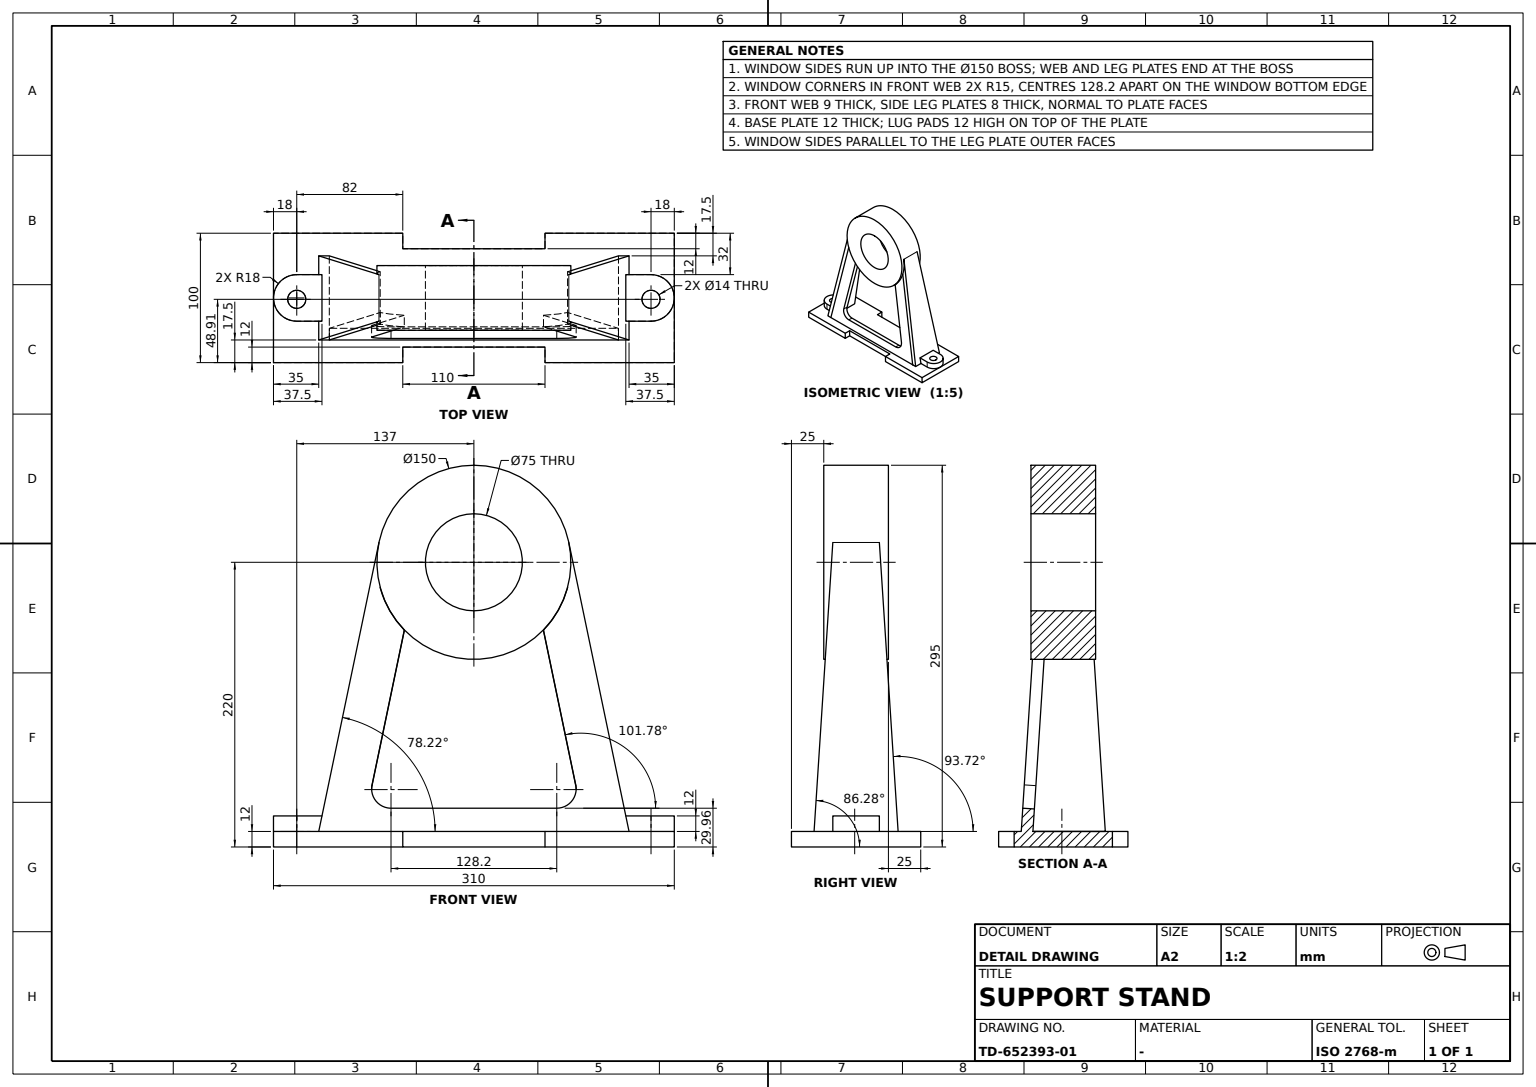
ISO-10303-21;
HEADER;
FILE_DESCRIPTION((''),'2;1');
FILE_NAME('','',(''),(''),'','','');
FILE_SCHEMA(('AUTOMOTIVE_DESIGN'));
ENDSEC;
DATA;
#1=APPLICATION_CONTEXT('');
#2=PRODUCT_CONTEXT('',#1,'mechanical');
#3=PRODUCT('','','',(#2));
#4=PRODUCT_DEFINITION_FORMATION('','',#3);
#5=PRODUCT_DEFINITION_CONTEXT('',#1,'design');
#6=PRODUCT_DEFINITION('','',#4,#5);
#7=PRODUCT_DEFINITION_SHAPE('','',#6);
#8=(LENGTH_UNIT()NAMED_UNIT(*)SI_UNIT(.MILLI.,.METRE.));
#9=(NAMED_UNIT(*)PLANE_ANGLE_UNIT()SI_UNIT($,.RADIAN.));
#10=(NAMED_UNIT(*)SI_UNIT($,.STERADIAN.)SOLID_ANGLE_UNIT());
#11=UNCERTAINTY_MEASURE_WITH_UNIT(LENGTH_MEASURE(0.005),#8,'distance_accuracy_value','');
#12=(GEOMETRIC_REPRESENTATION_CONTEXT(3)GLOBAL_UNCERTAINTY_ASSIGNED_CONTEXT((#11))GLOBAL_UNIT_ASSIGNED_CONTEXT((#8,#9,#10))REPRESENTATION_CONTEXT('',''));
#13=CARTESIAN_POINT('',(120.,32.5,0.));
#14=VERTEX_POINT('',#13);
#15=CARTESIAN_POINT('',(111.827821,32.5,0.));
#16=VERTEX_POINT('',#15);
#17=CARTESIAN_POINT('',(0.,32.5,0.));
#18=DIRECTION('',(-1.,0.,0.));
#19=VECTOR('',#18,1000.);
#20=LINE('',#17,#19);
#21=EDGE_CURVE('',#14,#16,#20,.T.);
#22=ORIENTED_EDGE('',*,*,#21,.F.);
#23=CARTESIAN_POINT('',(120.,18.,0.));
#24=VERTEX_POINT('',#23);
#25=CARTESIAN_POINT('',(120.,0.,0.));
#26=DIRECTION('',(0.,1.,0.));
#27=VECTOR('',#26,1000.);
#28=LINE('',#25,#27);
#29=EDGE_CURVE('',#24,#14,#28,.T.);
#30=ORIENTED_EDGE('',*,*,#29,.F.);
#31=CARTESIAN_POINT('',(137.,18.,0.));
#32=VERTEX_POINT('',#31);
#33=LINE('',#31,#19);
#34=EDGE_CURVE('',#32,#24,#33,.T.);
#35=ORIENTED_EDGE('',*,*,#34,.F.);
#36=CARTESIAN_POINT('',(155.,0.,0.));
#37=VERTEX_POINT('',#36);
#38=CARTESIAN_POINT('',(137.,0.,0.));
#39=DIRECTION('',(0.,0.,-1.));
#40=AXIS2_PLACEMENT_3D('',#38,#39,#18);
#41=CIRCLE('',#40,18.);
#42=EDGE_CURVE('',#37,#32,#41,.F.);
#43=ORIENTED_EDGE('',*,*,#42,.F.);
#44=CARTESIAN_POINT('',(155.,50.,0.));
#45=VERTEX_POINT('',#44);
#46=DIRECTION('',(0.,-1.,0.));
#47=VECTOR('',#46,1000.);
#48=LINE('',#36,#47);
#49=EDGE_CURVE('',#45,#37,#48,.T.);
#50=ORIENTED_EDGE('',*,*,#49,.F.);
#51=CARTESIAN_POINT('',(55.,50.,0.));
#52=VERTEX_POINT('',#51);
#53=CARTESIAN_POINT('',(0.,50.,0.));
#54=DIRECTION('',(1.,0.,0.));
#55=VECTOR('',#54,1000.);
#56=LINE('',#53,#55);
#57=EDGE_CURVE('',#52,#45,#56,.T.);
#58=ORIENTED_EDGE('',*,*,#57,.F.);
#59=CARTESIAN_POINT('',(55.,38.,0.));
#60=VERTEX_POINT('',#59);
#61=CARTESIAN_POINT('',(55.,0.,0.));
#62=LINE('',#61,#27);
#63=EDGE_CURVE('',#60,#52,#62,.T.);
#64=ORIENTED_EDGE('',*,*,#63,.F.);
#65=CARTESIAN_POINT('',(-55.,38.,0.));
#66=VERTEX_POINT('',#65);
#67=CARTESIAN_POINT('',(0.,38.,0.));
#68=LINE('',#67,#55);
#69=EDGE_CURVE('',#66,#60,#68,.T.);
#70=ORIENTED_EDGE('',*,*,#69,.F.);
#71=CARTESIAN_POINT('',(-55.,50.,0.));
#72=VERTEX_POINT('',#71);
#73=CARTESIAN_POINT('',(-55.,0.,0.));
#74=LINE('',#73,#47);
#75=EDGE_CURVE('',#72,#66,#74,.T.);
#76=ORIENTED_EDGE('',*,*,#75,.F.);
#77=CARTESIAN_POINT('',(-155.,50.,0.));
#78=VERTEX_POINT('',#77);
#79=EDGE_CURVE('',#78,#72,#56,.T.);
#80=ORIENTED_EDGE('',*,*,#79,.F.);
#81=CARTESIAN_POINT('',(-155.,0.,0.));
#82=VERTEX_POINT('',#81);
#83=LINE('',#81,#27);
#84=EDGE_CURVE('',#82,#78,#83,.T.);
#85=ORIENTED_EDGE('',*,*,#84,.F.);
#86=CARTESIAN_POINT('',(-137.,18.,0.));
#87=VERTEX_POINT('',#86);
#88=CARTESIAN_POINT('',(-137.,0.,0.));
#89=AXIS2_PLACEMENT_3D('',#88,#39,#18);
#90=CIRCLE('',#89,18.);
#91=EDGE_CURVE('',#82,#87,#90,.T.);
#92=ORIENTED_EDGE('',*,*,#91,.T.);
#93=CARTESIAN_POINT('',(-120.,18.,0.));
#94=VERTEX_POINT('',#93);
#95=CARTESIAN_POINT('',(0.,18.,0.));
#96=LINE('',#95,#55);
#97=EDGE_CURVE('',#87,#94,#96,.T.);
#98=ORIENTED_EDGE('',*,*,#97,.T.);
#99=CARTESIAN_POINT('',(-120.,32.5,0.));
#100=VERTEX_POINT('',#99);
#101=CARTESIAN_POINT('',(-120.,0.,0.));
#102=LINE('',#101,#27);
#103=EDGE_CURVE('',#94,#100,#102,.T.);
#104=ORIENTED_EDGE('',*,*,#103,.T.);
#105=CARTESIAN_POINT('',(-111.827821,32.5,0.));
#106=VERTEX_POINT('',#105);
#107=EDGE_CURVE('',#106,#100,#20,.T.);
#108=ORIENTED_EDGE('',*,*,#107,.F.);
#109=CARTESIAN_POINT('',(-111.827821,-32.5,0.));
#110=VERTEX_POINT('',#109);
#111=CARTESIAN_POINT('',(-111.827821,0.,0.));
#112=LINE('',#111,#47);
#113=EDGE_CURVE('',#106,#110,#112,.T.);
#114=ORIENTED_EDGE('',*,*,#113,.T.);
#115=CARTESIAN_POINT('',(-111.706184,-23.481048,0.));
#116=VERTEX_POINT('',#115);
#117=CARTESIAN_POINT('',(-111.369243,1.502014,0.));
#118=DIRECTION('',(0.013485569,0.999909066,0.));
#119=VECTOR('',#118,1000.);
#120=LINE('',#117,#119);
#121=EDGE_CURVE('',#110,#116,#120,.T.);
#122=ORIENTED_EDGE('',*,*,#121,.T.);
#123=CARTESIAN_POINT('',(111.706184,-23.481048,0.));
#124=VERTEX_POINT('',#123);
#125=CARTESIAN_POINT('',(0.,-23.481048,0.));
#126=LINE('',#125,#55);
#127=EDGE_CURVE('',#116,#124,#126,.T.);
#128=ORIENTED_EDGE('',*,*,#127,.T.);
#129=CARTESIAN_POINT('',(111.827821,-32.5,0.));
#130=VERTEX_POINT('',#129);
#131=CARTESIAN_POINT('',(111.369243,1.502014,0.));
#132=DIRECTION('',(-0.013485569,0.999909066,0.));
#133=VECTOR('',#132,1000.);
#134=LINE('',#131,#133);
#135=EDGE_CURVE('',#130,#124,#134,.T.);
#136=ORIENTED_EDGE('',*,*,#135,.F.);
#137=CARTESIAN_POINT('',(111.827821,0.,0.));
#138=LINE('',#137,#47);
#139=EDGE_CURVE('',#16,#130,#138,.T.);
#140=ORIENTED_EDGE('',*,*,#139,.F.);
#141=EDGE_LOOP('',(#22,#30,#35,#43,#50,#58,#64,#70,#76,#80,#85,#92,#98,#104,#108,#114,#122,#128,#136,#140));
#142=FACE_BOUND('',#141,.T.);
#143=CARTESIAN_POINT('',(0.,0.,0.));
#144=AXIS2_PLACEMENT_3D('',#143,#39,#18);
#145=PLANE('',#144);
#146=ADVANCED_FACE('',(#142),#145,.F.);
#147=CARTESIAN_POINT('',(-137.,-18.,12.));
#148=VERTEX_POINT('',#147);
#149=CARTESIAN_POINT('',(-137.,18.,12.));
#150=VERTEX_POINT('',#149);
#151=CARTESIAN_POINT('',(-137.,0.,12.));
#152=DIRECTION('',(0.,0.,1.));
#153=AXIS2_PLACEMENT_3D('',#151,#152,#54);
#154=CIRCLE('',#153,18.);
#155=EDGE_CURVE('',#148,#150,#154,.F.);
#156=ORIENTED_EDGE('',*,*,#155,.F.);
#157=CARTESIAN_POINT('',(-117.496972,-18.,12.));
#158=VERTEX_POINT('',#157);
#159=CARTESIAN_POINT('',(115.,-18.,12.));
#160=LINE('',#159,#19);
#161=EDGE_CURVE('',#158,#148,#160,.T.);
#162=ORIENTED_EDGE('',*,*,#161,.F.);
#163=CARTESIAN_POINT('',(-117.496972,18.,12.));
#164=VERTEX_POINT('',#163);
#165=CARTESIAN_POINT('',(-117.496972,0.,12.));
#166=LINE('',#165,#47);
#167=EDGE_CURVE('',#164,#158,#166,.T.);
#168=ORIENTED_EDGE('',*,*,#167,.F.);
#169=CARTESIAN_POINT('',(137.,18.,12.));
#170=LINE('',#169,#55);
#171=EDGE_CURVE('',#150,#164,#170,.T.);
#172=ORIENTED_EDGE('',*,*,#171,.F.);
#173=EDGE_LOOP('',(#156,#162,#168,#172));
#174=FACE_BOUND('',#173,.T.);
#175=CARTESIAN_POINT('',(-130.,-1.086869,12.));
#176=VERTEX_POINT('',#175);
#177=CARTESIAN_POINT('',(-137.,-1.086869,12.));
#178=AXIS2_PLACEMENT_3D('',#177,#152,#54);
#179=CIRCLE('',#178,7.);
#180=EDGE_CURVE('',#176,#176,#179,.T.);
#181=ORIENTED_EDGE('',*,*,#180,.F.);
#182=EDGE_LOOP('',(#181));
#183=FACE_BOUND('',#182,.T.);
#184=CARTESIAN_POINT('',(0.,0.,12.));
#185=AXIS2_PLACEMENT_3D('',#184,#152,#46);
#186=PLANE('',#185);
#187=ADVANCED_FACE('',(#174,#183),#186,.T.);
#188=CARTESIAN_POINT('',(55.,-38.,0.));
#189=VERTEX_POINT('',#188);
#190=CARTESIAN_POINT('',(-55.,-38.,0.));
#191=VERTEX_POINT('',#190);
#192=CARTESIAN_POINT('',(0.,-38.,0.));
#193=LINE('',#192,#19);
#194=EDGE_CURVE('',#189,#191,#193,.T.);
#195=ORIENTED_EDGE('',*,*,#194,.T.);
#196=CARTESIAN_POINT('',(-55.,-38.,-12.));
#197=VERTEX_POINT('',#196);
#198=VECTOR('',#39,1000.);
#199=LINE('',#190,#198);
#200=EDGE_CURVE('',#191,#197,#199,.T.);
#201=ORIENTED_EDGE('',*,*,#200,.T.);
#202=CARTESIAN_POINT('',(55.,-38.,-12.));
#203=VERTEX_POINT('',#202);
#204=CARTESIAN_POINT('',(0.,-38.,-12.));
#205=LINE('',#204,#19);
#206=EDGE_CURVE('',#203,#197,#205,.T.);
#207=ORIENTED_EDGE('',*,*,#206,.F.);
#208=LINE('',#188,#198);
#209=EDGE_CURVE('',#189,#203,#208,.T.);
#210=ORIENTED_EDGE('',*,*,#209,.F.);
#211=EDGE_LOOP('',(#195,#201,#207,#210));
#212=FACE_BOUND('',#211,.T.);
#213=AXIS2_PLACEMENT_3D('',#188,#46,#18);
#214=PLANE('',#213);
#215=ADVANCED_FACE('',(#212),#214,.T.);
#216=CARTESIAN_POINT('',(144.,-1.086869,12.));
#217=VERTEX_POINT('',#216);
#218=CARTESIAN_POINT('',(137.,-1.086869,12.));
#219=AXIS2_PLACEMENT_3D('',#218,#152,#54);
#220=CIRCLE('',#219,7.);
#221=EDGE_CURVE('',#217,#217,#220,.T.);
#222=ORIENTED_EDGE('',*,*,#221,.T.);
#223=EDGE_LOOP('',(#222));
#224=FACE_BOUND('',#223,.T.);
#225=CARTESIAN_POINT('',(130.,-1.086869,-12.));
#226=VERTEX_POINT('',#225);
#227=CARTESIAN_POINT('',(137.,-1.086869,-12.));
#228=AXIS2_PLACEMENT_3D('',#227,#39,#18);
#229=CIRCLE('',#228,7.);
#230=EDGE_CURVE('',#226,#226,#229,.T.);
#231=ORIENTED_EDGE('',*,*,#230,.T.);
#232=EDGE_LOOP('',(#231));
#233=FACE_BOUND('',#232,.T.);
#234=CARTESIAN_POINT('',(137.,-1.086869,11.9));
#235=AXIS2_PLACEMENT_3D('',#234,#39,#54);
#236=CYLINDRICAL_SURFACE('',#235,7.);
#237=ADVANCED_FACE('',(#224,#233),#236,.F.);
#238=CARTESIAN_POINT('',(120.,-18.,0.));
#239=VERTEX_POINT('',#238);
#240=CARTESIAN_POINT('',(117.496972,-18.,12.));
#241=VERTEX_POINT('',#240);
#242=CARTESIAN_POINT('',(119.79153,-18.,0.999445));
#243=DIRECTION('',(-0.204191001,0.,0.978931068));
#244=VECTOR('',#243,1000.);
#245=LINE('',#242,#244);
#246=EDGE_CURVE('',#239,#241,#245,.T.);
#247=ORIENTED_EDGE('',*,*,#246,.F.);
#248=CARTESIAN_POINT('',(137.,-18.,0.));
#249=VERTEX_POINT('',#248);
#250=CARTESIAN_POINT('',(115.,-18.,0.));
#251=LINE('',#250,#55);
#252=EDGE_CURVE('',#239,#249,#251,.T.);
#253=ORIENTED_EDGE('',*,*,#252,.T.);
#254=CARTESIAN_POINT('',(137.,-18.,12.));
#255=VERTEX_POINT('',#254);
#256=CARTESIAN_POINT('',(137.,-18.,6.));
#257=VECTOR('',#152,1000.);
#258=LINE('',#256,#257);
#259=EDGE_CURVE('',#249,#255,#258,.T.);
#260=ORIENTED_EDGE('',*,*,#259,.T.);
#261=CARTESIAN_POINT('',(0.,-18.,12.));
#262=LINE('',#261,#55);
#263=EDGE_CURVE('',#241,#255,#262,.T.);
#264=ORIENTED_EDGE('',*,*,#263,.F.);
#265=EDGE_LOOP('',(#247,#253,#260,#264));
#266=FACE_BOUND('',#265,.T.);
#267=AXIS2_PLACEMENT_3D('',#250,#46,#54);
#268=PLANE('',#267);
#269=ADVANCED_FACE('',(#266),#268,.T.);
#270=CARTESIAN_POINT('',(120.,-32.5,0.));
#271=VERTEX_POINT('',#270);
#272=CARTESIAN_POINT('',(73.41983,-18.,223.314325));
#273=VERTEX_POINT('',#272);
#274=CARTESIAN_POINT('',(115.016857,-30.948791,23.890148));
#275=DIRECTION('',(-0.203779756,0.063434858,0.976959482));
#276=VECTOR('',#275,1000.);
#277=LINE('',#274,#276);
#278=EDGE_CURVE('',#271,#273,#277,.T.);
#279=ORIENTED_EDGE('',*,*,#278,.F.);
#280=EDGE_CURVE('',#271,#239,#28,.T.);
#281=ORIENTED_EDGE('',*,*,#280,.T.);
#282=ORIENTED_EDGE('',*,*,#246,.T.);
#283=CARTESIAN_POINT('',(117.496972,18.,12.));
#284=VERTEX_POINT('',#283);
#285=CARTESIAN_POINT('',(117.496972,0.,12.));
#286=LINE('',#285,#47);
#287=EDGE_CURVE('',#284,#241,#286,.T.);
#288=ORIENTED_EDGE('',*,*,#287,.F.);
#289=CARTESIAN_POINT('',(73.41983,18.,223.314325));
#290=LINE('',#289,#244);
#291=EDGE_CURVE('',#24,#284,#290,.T.);
#292=ORIENTED_EDGE('',*,*,#291,.F.);
#293=ORIENTED_EDGE('',*,*,#29,.T.);
#294=VERTEX_POINT('',#289);
#295=CARTESIAN_POINT('',(115.016857,30.948791,23.890148));
#296=DIRECTION('',(-0.203779756,-0.063434858,0.976959482));
#297=VECTOR('',#296,1000.);
#298=LINE('',#295,#297);
#299=EDGE_CURVE('',#14,#294,#298,.T.);
#300=ORIENTED_EDGE('',*,*,#299,.T.);
#301=CARTESIAN_POINT('',(73.41983,0.,223.314325));
#302=LINE('',#301,#27);
#303=EDGE_CURVE('',#273,#294,#302,.T.);
#304=ORIENTED_EDGE('',*,*,#303,.F.);
#305=EDGE_LOOP('',(#279,#281,#282,#288,#292,#293,#300,#304));
#306=FACE_BOUND('',#305,.T.);
#307=DIRECTION('',(0.978931068,0.,0.204191001));
#308=DIRECTION('',(0.204191001,0.,-0.978931068));
#309=AXIS2_PLACEMENT_3D('',#301,#307,#308);
#310=PLANE('',#309);
#311=ADVANCED_FACE('',(#306),#310,.T.);
#312=ORIENTED_EDGE('',*,*,#263,.T.);
#313=VERTEX_POINT('',#169);
#314=CARTESIAN_POINT('',(137.,0.,12.));
#315=AXIS2_PLACEMENT_3D('',#314,#152,#54);
#316=CIRCLE('',#315,18.);
#317=EDGE_CURVE('',#255,#313,#316,.T.);
#318=ORIENTED_EDGE('',*,*,#317,.T.);
#319=CARTESIAN_POINT('',(0.,18.,12.));
#320=LINE('',#319,#19);
#321=EDGE_CURVE('',#313,#284,#320,.T.);
#322=ORIENTED_EDGE('',*,*,#321,.T.);
#323=ORIENTED_EDGE('',*,*,#287,.T.);
#324=EDGE_LOOP('',(#312,#318,#322,#323));
#325=FACE_BOUND('',#324,.T.);
#326=ORIENTED_EDGE('',*,*,#221,.F.);
#327=EDGE_LOOP('',(#326));
#328=FACE_BOUND('',#327,.T.);
#329=ADVANCED_FACE('',(#325,#328),#186,.T.);
#330=ORIENTED_EDGE('',*,*,#180,.T.);
#331=EDGE_LOOP('',(#330));
#332=FACE_BOUND('',#331,.T.);
#333=CARTESIAN_POINT('',(-144.,-1.086869,-12.));
#334=VERTEX_POINT('',#333);
#335=CARTESIAN_POINT('',(-137.,-1.086869,-12.));
#336=AXIS2_PLACEMENT_3D('',#335,#39,#18);
#337=CIRCLE('',#336,7.);
#338=EDGE_CURVE('',#334,#334,#337,.T.);
#339=ORIENTED_EDGE('',*,*,#338,.T.);
#340=EDGE_LOOP('',(#339));
#341=FACE_BOUND('',#340,.T.);
#342=CARTESIAN_POINT('',(-137.,-1.086869,11.9));
#343=AXIS2_PLACEMENT_3D('',#342,#39,#54);
#344=CYLINDRICAL_SURFACE('',#343,7.);
#345=ADVANCED_FACE('',(#332,#341),#344,.F.);
#346=CARTESIAN_POINT('',(0.,25.,283.));
#347=VERTEX_POINT('',#346);
#348=CARTESIAN_POINT('',(0.,25.,208.));
#349=AXIS2_PLACEMENT_3D('',#348,#26,#152);
#350=CIRCLE('',#349,75.);
#351=EDGE_CURVE('',#347,#347,#350,.T.);
#352=ORIENTED_EDGE('',*,*,#351,.T.);
#353=EDGE_LOOP('',(#352));
#354=FACE_BOUND('',#353,.T.);
#355=CARTESIAN_POINT('',(0.,25.,245.5));
#356=VERTEX_POINT('',#355);
#357=CIRCLE('',#349,37.5);
#358=EDGE_CURVE('',#356,#356,#357,.T.);
#359=ORIENTED_EDGE('',*,*,#358,.F.);
#360=EDGE_LOOP('',(#359));
#361=FACE_BOUND('',#360,.T.);
#362=CARTESIAN_POINT('',(0.,25.,0.));
#363=AXIS2_PLACEMENT_3D('',#362,#26,#18);
#364=PLANE('',#363);
#365=ADVANCED_FACE('',(#354,#361),#364,.T.);
#366=CARTESIAN_POINT('',(-72.506512,-20.25962,188.513943));
#367=VERTEX_POINT('',#366);
#368=DIRECTION('',(0.203779756,0.063434858,0.976959482));
#369=VECTOR('',#368,1000.);
#370=LINE('',#109,#369);
#371=EDGE_CURVE('',#110,#367,#370,.T.);
#372=ORIENTED_EDGE('',*,*,#371,.F.);
#373=ORIENTED_EDGE('',*,*,#113,.F.);
#374=CARTESIAN_POINT('',(-72.470557,20.248428,188.686318));
#375=VERTEX_POINT('',#374);
#376=CARTESIAN_POINT('',(-65.01497,17.927568,224.429844));
#377=DIRECTION('',(0.203779756,-0.063434858,0.976959482));
#378=VECTOR('',#377,1000.);
#379=LINE('',#376,#378);
#380=EDGE_CURVE('',#106,#375,#379,.T.);
#381=ORIENTED_EDGE('',*,*,#380,.T.);
#382=CARTESIAN_POINT('',(-72.470557,-20.248428,188.686318));
#383=VERTEX_POINT('',#382);
#384=CARTESIAN_POINT('',(-72.470557,-20.248427,188.686318));
#385=LINE('',#384,#27);
#386=EDGE_CURVE('',#383,#375,#385,.T.);
#387=ORIENTED_EDGE('',*,*,#386,.F.);
#388=CARTESIAN_POINT('',(-65.01497,-17.927568,224.429844));
#389=LINE('',#388,#369);
#390=EDGE_CURVE('',#367,#383,#389,.T.);
#391=ORIENTED_EDGE('',*,*,#390,.F.);
#392=EDGE_LOOP('',(#372,#373,#381,#387,#391));
#393=FACE_BOUND('',#392,.T.);
#394=CARTESIAN_POINT('',(-65.247651,0.,223.314325));
#395=DIRECTION('',(-0.978931068,0.,0.204191001));
#396=DIRECTION('',(-0.204191001,0.,-0.978931068));
#397=AXIS2_PLACEMENT_3D('',#394,#395,#396);
#398=PLANE('',#397);
#399=ADVANCED_FACE('',(#393),#398,.F.);
#400=CARTESIAN_POINT('',(-73.41983,18.,223.314325));
#401=VERTEX_POINT('',#400);
#402=CARTESIAN_POINT('',(0.,18.994373,208.));
#403=DIRECTION('',(0.,-0.997898631,-0.064794456));
#404=DIRECTION('',(0.,0.064794456,-0.997898631));
#405=AXIS2_PLACEMENT_3D('',#402,#403,#404);
#406=ELLIPSE('',#405,75.157935,75.);
#407=EDGE_CURVE('',#375,#401,#406,.F.);
#408=ORIENTED_EDGE('',*,*,#407,.F.);
#409=ORIENTED_EDGE('',*,*,#380,.F.);
#410=ORIENTED_EDGE('',*,*,#107,.T.);
#411=CARTESIAN_POINT('',(-119.579881,32.369221,2.014132));
#412=LINE('',#411,#378);
#413=EDGE_CURVE('',#100,#401,#412,.T.);
#414=ORIENTED_EDGE('',*,*,#413,.T.);
#415=EDGE_LOOP('',(#408,#409,#410,#414));
#416=FACE_BOUND('',#415,.T.);
#417=DIRECTION('',(0.,-0.064794456,0.997898631));
#418=AXIS2_PLACEMENT_3D('',#17,#403,#417);
#419=PLANE('',#418);
#420=ADVANCED_FACE('',(#416),#419,.F.);
#421=CARTESIAN_POINT('',(-55.,38.,-12.));
#422=VERTEX_POINT('',#421);
#423=CARTESIAN_POINT('',(55.,38.,-12.));
#424=VERTEX_POINT('',#423);
#425=CARTESIAN_POINT('',(0.,38.,-12.));
#426=LINE('',#425,#55);
#427=EDGE_CURVE('',#422,#424,#426,.T.);
#428=ORIENTED_EDGE('',*,*,#427,.F.);
#429=LINE('',#65,#198);
#430=EDGE_CURVE('',#66,#422,#429,.T.);
#431=ORIENTED_EDGE('',*,*,#430,.F.);
#432=ORIENTED_EDGE('',*,*,#69,.T.);
#433=LINE('',#59,#198);
#434=EDGE_CURVE('',#60,#424,#433,.T.);
#435=ORIENTED_EDGE('',*,*,#434,.T.);
#436=EDGE_LOOP('',(#428,#431,#432,#435));
#437=FACE_BOUND('',#436,.T.);
#438=AXIS2_PLACEMENT_3D('',#65,#26,#54);
#439=PLANE('',#438);
#440=ADVANCED_FACE('',(#437),#439,.T.);
#441=CARTESIAN_POINT('',(64.101639,-22.352612,17.379025));
#442=VERTEX_POINT('',#441);
#443=CARTESIAN_POINT('',(-64.101639,-22.352612,17.379025));
#444=VERTEX_POINT('',#443);
#445=LINE('',#441,#19);
#446=EDGE_CURVE('',#442,#444,#445,.T.);
#447=ORIENTED_EDGE('',*,*,#446,.T.);
#448=CARTESIAN_POINT('',(-64.101639,-31.3337,17.962175));
#449=VERTEX_POINT('',#448);
#450=CARTESIAN_POINT('',(-64.101639,-26.843156,17.6706));
#451=DIRECTION('',(0.,-0.997898631,0.064794456));
#452=VECTOR('',#451,1000.);
#453=LINE('',#450,#452);
#454=EDGE_CURVE('',#449,#444,#453,.F.);
#455=ORIENTED_EDGE('',*,*,#454,.F.);
#456=CARTESIAN_POINT('',(64.101639,-31.3337,17.962175));
#457=VERTEX_POINT('',#456);
#458=LINE('',#456,#19);
#459=EDGE_CURVE('',#457,#449,#458,.T.);
#460=ORIENTED_EDGE('',*,*,#459,.F.);
#461=CARTESIAN_POINT('',(64.101639,-26.843156,17.6706));
#462=LINE('',#461,#452);
#463=EDGE_CURVE('',#457,#442,#462,.F.);
#464=ORIENTED_EDGE('',*,*,#463,.T.);
#465=EDGE_LOOP('',(#447,#455,#460,#464));
#466=FACE_BOUND('',#465,.T.);
#467=DIRECTION('',(0.,-0.064794456,-0.997898631));
#468=AXIS2_PLACEMENT_3D('',#456,#467,#18);
#469=PLANE('',#468);
#470=ADVANCED_FACE('',(#466),#469,.F.);
#471=CARTESIAN_POINT('',(55.,-50.,-12.));
#472=VERTEX_POINT('',#471);
#473=CARTESIAN_POINT('',(55.,0.,-12.));
#474=LINE('',#473,#27);
#475=EDGE_CURVE('',#472,#203,#474,.T.);
#476=ORIENTED_EDGE('',*,*,#475,.F.);
#477=CARTESIAN_POINT('',(55.,-50.,0.));
#478=VERTEX_POINT('',#477);
#479=LINE('',#477,#198);
#480=EDGE_CURVE('',#478,#472,#479,.T.);
#481=ORIENTED_EDGE('',*,*,#480,.F.);
#482=EDGE_CURVE('',#478,#189,#62,.T.);
#483=ORIENTED_EDGE('',*,*,#482,.T.);
#484=ORIENTED_EDGE('',*,*,#209,.T.);
#485=EDGE_LOOP('',(#476,#481,#483,#484));
#486=FACE_BOUND('',#485,.T.);
#487=AXIS2_PLACEMENT_3D('',#477,#18,#26);
#488=PLANE('',#487);
#489=ADVANCED_FACE('',(#486),#488,.T.);
#490=CARTESIAN_POINT('',(0.,-25.,245.5));
#491=VERTEX_POINT('',#490);
#492=CARTESIAN_POINT('',(0.,-25.,208.));
#493=AXIS2_PLACEMENT_3D('',#492,#26,#152);
#494=CIRCLE('',#493,37.5);
#495=EDGE_CURVE('',#491,#491,#494,.T.);
#496=ORIENTED_EDGE('',*,*,#495,.T.);
#497=EDGE_LOOP('',(#496));
#498=FACE_BOUND('',#497,.T.);
#499=CARTESIAN_POINT('',(0.,-25.,283.));
#500=VERTEX_POINT('',#499);
#501=CIRCLE('',#493,75.);
#502=EDGE_CURVE('',#500,#500,#501,.T.);
#503=ORIENTED_EDGE('',*,*,#502,.F.);
#504=EDGE_LOOP('',(#503));
#505=FACE_BOUND('',#504,.T.);
#506=CARTESIAN_POINT('',(0.,-25.,0.));
#507=AXIS2_PLACEMENT_3D('',#506,#26,#18);
#508=PLANE('',#507);
#509=ADVANCED_FACE('',(#498,#505),#508,.F.);
#510=CARTESIAN_POINT('',(-78.78689,-30.163726,35.980928));
#511=VERTEX_POINT('',#510);
#512=CARTESIAN_POINT('',(-53.833779,-22.39604,155.610962));
#513=VERTEX_POINT('',#512);
#514=LINE('',#510,#369);
#515=EDGE_CURVE('',#511,#513,#514,.T.);
#516=ORIENTED_EDGE('',*,*,#515,.T.);
#517=CARTESIAN_POINT('',(-62.739025,-21.802448,164.752876));
#518=CARTESIAN_POINT('',(-69.235978,-21.059106,176.201073));
#519=B_SPLINE_CURVE_WITH_KNOTS('',3,(#512,#517,#518,#366),.UNSPECIFIED.,.F.,.F.,(4,4),(0.25858219,0.770182356),.UNSPECIFIED.);
#520=EDGE_CURVE('',#367,#513,#519,.F.);
#521=ORIENTED_EDGE('',*,*,#520,.F.);
#522=ORIENTED_EDGE('',*,*,#390,.T.);
#523=CARTESIAN_POINT('',(-73.41983,-18.,223.314325));
#524=VERTEX_POINT('',#523);
#525=CARTESIAN_POINT('',(0.,-18.994373,208.));
#526=DIRECTION('',(0.,0.064794456,0.997898631));
#527=AXIS2_PLACEMENT_3D('',#525,#451,#526);
#528=ELLIPSE('',#527,75.157935,75.);
#529=EDGE_CURVE('',#383,#524,#528,.F.);
#530=ORIENTED_EDGE('',*,*,#529,.T.);
#531=CARTESIAN_POINT('',(-120.,-32.5,0.));
#532=VERTEX_POINT('',#531);
#533=CARTESIAN_POINT('',(-119.579881,-32.369221,2.014132));
#534=LINE('',#533,#369);
#535=EDGE_CURVE('',#532,#524,#534,.T.);
#536=ORIENTED_EDGE('',*,*,#535,.F.);
#537=CARTESIAN_POINT('',(0.,-32.5,0.));
#538=LINE('',#537,#55);
#539=EDGE_CURVE('',#532,#271,#538,.T.);
#540=ORIENTED_EDGE('',*,*,#539,.T.);
#541=ORIENTED_EDGE('',*,*,#278,.T.);
#542=CARTESIAN_POINT('',(72.470557,-20.248428,188.686318));
#543=VERTEX_POINT('',#542);
#544=EDGE_CURVE('',#273,#543,#528,.F.);
#545=ORIENTED_EDGE('',*,*,#544,.T.);
#546=CARTESIAN_POINT('',(72.506512,-20.25962,188.513943));
#547=VERTEX_POINT('',#546);
#548=CARTESIAN_POINT('',(107.184038,-31.054431,22.263193));
#549=LINE('',#548,#276);
#550=EDGE_CURVE('',#547,#543,#549,.T.);
#551=ORIENTED_EDGE('',*,*,#550,.F.);
#552=CARTESIAN_POINT('',(53.833779,-22.39604,155.610962));
#553=VERTEX_POINT('',#552);
#554=CARTESIAN_POINT('',(69.235978,-21.059106,176.201073));
#555=CARTESIAN_POINT('',(62.739025,-21.802448,164.752876));
#556=B_SPLINE_CURVE_WITH_KNOTS('',3,(#546,#554,#555,#552),.UNSPECIFIED.,.F.,.F.,(4,4),(2.371410298,2.883010464),.UNSPECIFIED.);
#557=EDGE_CURVE('',#553,#547,#556,.F.);
#558=ORIENTED_EDGE('',*,*,#557,.F.);
#559=CARTESIAN_POINT('',(78.78689,-30.163726,35.980928));
#560=VERTEX_POINT('',#559);
#561=DIRECTION('',(0.203779756,-0.063434858,-0.976959482));
#562=VECTOR('',#561,1000.);
#563=LINE('',#552,#562);
#564=EDGE_CURVE('',#553,#560,#563,.T.);
#565=ORIENTED_EDGE('',*,*,#564,.T.);
#566=CARTESIAN_POINT('',(64.101639,-30.361783,32.930655));
#567=AXIS2_PLACEMENT_3D('',#566,#451,#467);
#568=CIRCLE('',#567,15.);
#569=EDGE_CURVE('',#457,#560,#568,.T.);
#570=ORIENTED_EDGE('',*,*,#569,.F.);
#571=ORIENTED_EDGE('',*,*,#459,.T.);
#572=CARTESIAN_POINT('',(-64.101639,-30.361783,32.930655));
#573=AXIS2_PLACEMENT_3D('',#572,#451,#467);
#574=CIRCLE('',#573,15.);
#575=EDGE_CURVE('',#511,#449,#574,.T.);
#576=ORIENTED_EDGE('',*,*,#575,.F.);
#577=EDGE_LOOP('',(#516,#521,#522,#530,#536,#540,#541,#545,#551,#558,#565,#570,#571,#576));
#578=FACE_BOUND('',#577,.T.);
#579=AXIS2_PLACEMENT_3D('',#537,#451,#526);
#580=PLANE('',#579);
#581=ADVANCED_FACE('',(#578),#580,.T.);
#582=ORIENTED_EDGE('',*,*,#529,.F.);
#583=ORIENTED_EDGE('',*,*,#386,.T.);
#584=ORIENTED_EDGE('',*,*,#407,.T.);
#585=CARTESIAN_POINT('',(-73.41983,0.,223.314325));
#586=LINE('',#585,#27);
#587=EDGE_CURVE('',#524,#401,#586,.T.);
#588=ORIENTED_EDGE('',*,*,#587,.F.);
#589=EDGE_LOOP('',(#582,#583,#584,#588));
#590=FACE_BOUND('',#589,.T.);
#591=ORIENTED_EDGE('',*,*,#351,.F.);
#592=EDGE_LOOP('',(#591));
#593=FACE_BOUND('',#592,.T.);
#594=ORIENTED_EDGE('',*,*,#303,.T.);
#595=CARTESIAN_POINT('',(72.470557,20.248428,188.686318));
#596=VERTEX_POINT('',#595);
#597=EDGE_CURVE('',#294,#596,#406,.F.);
#598=ORIENTED_EDGE('',*,*,#597,.T.);
#599=CARTESIAN_POINT('',(72.470557,-20.248427,188.686318));
#600=LINE('',#599,#27);
#601=EDGE_CURVE('',#543,#596,#600,.T.);
#602=ORIENTED_EDGE('',*,*,#601,.F.);
#603=ORIENTED_EDGE('',*,*,#544,.F.);
#604=EDGE_LOOP('',(#594,#598,#602,#603));
#605=FACE_BOUND('',#604,.T.);
#606=ORIENTED_EDGE('',*,*,#502,.T.);
#607=EDGE_LOOP('',(#606));
#608=FACE_BOUND('',#607,.T.);
#609=CARTESIAN_POINT('',(0.,0.,208.));
#610=AXIS2_PLACEMENT_3D('',#609,#26,#18);
#611=CYLINDRICAL_SURFACE('',#610,75.);
#612=ADVANCED_FACE('',(#590,#593,#605,#608),#611,.T.);
#613=CARTESIAN_POINT('',(-55.,-50.,0.));
#614=VERTEX_POINT('',#613);
#615=CARTESIAN_POINT('',(-55.,-50.,-12.));
#616=VERTEX_POINT('',#615);
#617=LINE('',#613,#198);
#618=EDGE_CURVE('',#614,#616,#617,.T.);
#619=ORIENTED_EDGE('',*,*,#618,.F.);
#620=CARTESIAN_POINT('',(-155.,-50.,0.));
#621=VERTEX_POINT('',#620);
#622=CARTESIAN_POINT('',(0.,-50.,0.));
#623=LINE('',#622,#19);
#624=EDGE_CURVE('',#614,#621,#623,.T.);
#625=ORIENTED_EDGE('',*,*,#624,.T.);
#626=CARTESIAN_POINT('',(-155.,-50.,-12.));
#627=VERTEX_POINT('',#626);
#628=LINE('',#620,#198);
#629=EDGE_CURVE('',#621,#627,#628,.T.);
#630=ORIENTED_EDGE('',*,*,#629,.T.);
#631=CARTESIAN_POINT('',(0.,-50.,-12.));
#632=LINE('',#631,#19);
#633=EDGE_CURVE('',#616,#627,#632,.T.);
#634=ORIENTED_EDGE('',*,*,#633,.F.);
#635=EDGE_LOOP('',(#619,#625,#630,#634));
#636=FACE_BOUND('',#635,.T.);
#637=CARTESIAN_POINT('',(155.,-50.,0.));
#638=AXIS2_PLACEMENT_3D('',#637,#46,#18);
#639=PLANE('',#638);
#640=ADVANCED_FACE('',(#636),#639,.T.);
#641=ORIENTED_EDGE('',*,*,#495,.F.);
#642=EDGE_LOOP('',(#641));
#643=FACE_BOUND('',#642,.T.);
#644=ORIENTED_EDGE('',*,*,#358,.T.);
#645=EDGE_LOOP('',(#644));
#646=FACE_BOUND('',#645,.T.);
#647=CYLINDRICAL_SURFACE('',#610,37.5);
#648=ADVANCED_FACE('',(#643,#646),#647,.F.);
#649=ORIENTED_EDGE('',*,*,#569,.T.);
#650=CARTESIAN_POINT('',(78.78689,-21.182638,35.397778));
#651=VERTEX_POINT('',#650);
#652=CARTESIAN_POINT('',(78.78689,-25.673182,35.689353));
#653=LINE('',#652,#452);
#654=EDGE_CURVE('',#560,#651,#653,.F.);
#655=ORIENTED_EDGE('',*,*,#654,.T.);
#656=CARTESIAN_POINT('',(64.101639,-21.380695,32.347505));
#657=AXIS2_PLACEMENT_3D('',#656,#451,#467);
#658=CIRCLE('',#657,15.);
#659=EDGE_CURVE('',#442,#651,#658,.T.);
#660=ORIENTED_EDGE('',*,*,#659,.F.);
#661=ORIENTED_EDGE('',*,*,#463,.F.);
#662=EDGE_LOOP('',(#649,#655,#660,#661));
#663=FACE_BOUND('',#662,.T.);
#664=CARTESIAN_POINT('',(64.101639,-25.871239,32.63908));
#665=AXIS2_PLACEMENT_3D('',#664,#451,#54);
#666=CYLINDRICAL_SURFACE('',#665,15.);
#667=ADVANCED_FACE('',(#663),#666,.F.);
#668=VERTEX_POINT('',#637);
#669=CARTESIAN_POINT('',(155.,-50.,-12.));
#670=VERTEX_POINT('',#669);
#671=LINE('',#637,#198);
#672=EDGE_CURVE('',#668,#670,#671,.T.);
#673=ORIENTED_EDGE('',*,*,#672,.T.);
#674=CARTESIAN_POINT('',(155.,50.,-12.));
#675=VERTEX_POINT('',#674);
#676=CARTESIAN_POINT('',(155.,0.,-12.));
#677=LINE('',#676,#47);
#678=EDGE_CURVE('',#675,#670,#677,.T.);
#679=ORIENTED_EDGE('',*,*,#678,.F.);
#680=LINE('',#44,#198);
#681=EDGE_CURVE('',#45,#675,#680,.T.);
#682=ORIENTED_EDGE('',*,*,#681,.F.);
#683=ORIENTED_EDGE('',*,*,#49,.T.);
#684=EDGE_CURVE('',#37,#668,#48,.T.);
#685=ORIENTED_EDGE('',*,*,#684,.T.);
#686=EDGE_LOOP('',(#673,#679,#682,#683,#685));
#687=FACE_BOUND('',#686,.T.);
#688=AXIS2_PLACEMENT_3D('',#44,#54,#46);
#689=PLANE('',#688);
#690=ADVANCED_FACE('',(#687),#689,.T.);
#691=EDGE_CURVE('',#191,#614,#74,.T.);
#692=ORIENTED_EDGE('',*,*,#691,.F.);
#693=ORIENTED_EDGE('',*,*,#194,.F.);
#694=ORIENTED_EDGE('',*,*,#482,.F.);
#695=EDGE_CURVE('',#668,#478,#623,.T.);
#696=ORIENTED_EDGE('',*,*,#695,.F.);
#697=ORIENTED_EDGE('',*,*,#684,.F.);
#698=EDGE_CURVE('',#249,#37,#41,.F.);
#699=ORIENTED_EDGE('',*,*,#698,.F.);
#700=ORIENTED_EDGE('',*,*,#252,.F.);
#701=ORIENTED_EDGE('',*,*,#280,.F.);
#702=ORIENTED_EDGE('',*,*,#539,.F.);
#703=CARTESIAN_POINT('',(-120.,-18.,0.));
#704=VERTEX_POINT('',#703);
#705=EDGE_CURVE('',#532,#704,#102,.T.);
#706=ORIENTED_EDGE('',*,*,#705,.T.);
#707=CARTESIAN_POINT('',(-137.,-18.,0.));
#708=VERTEX_POINT('',#707);
#709=CARTESIAN_POINT('',(0.,-18.,0.));
#710=LINE('',#709,#19);
#711=EDGE_CURVE('',#704,#708,#710,.T.);
#712=ORIENTED_EDGE('',*,*,#711,.T.);
#713=EDGE_CURVE('',#708,#82,#90,.T.);
#714=ORIENTED_EDGE('',*,*,#713,.T.);
#715=EDGE_CURVE('',#621,#82,#83,.T.);
#716=ORIENTED_EDGE('',*,*,#715,.F.);
#717=ORIENTED_EDGE('',*,*,#624,.F.);
#718=EDGE_LOOP('',(#692,#693,#694,#696,#697,#699,#700,#701,#702,#706,#712,#714,#716,#717));
#719=FACE_BOUND('',#718,.T.);
#720=ADVANCED_FACE('',(#719),#145,.F.);
#721=ORIENTED_EDGE('',*,*,#135,.T.);
#722=CARTESIAN_POINT('',(72.506512,-11.278532,187.930793));
#723=VERTEX_POINT('',#722);
#724=CARTESIAN_POINT('',(111.827821,-23.518912,-0.58315));
#725=LINE('',#724,#276);
#726=EDGE_CURVE('',#124,#723,#725,.T.);
#727=ORIENTED_EDGE('',*,*,#726,.T.);
#728=DIRECTION('',(0.,0.997898631,-0.064794456));
#729=VECTOR('',#728,1000.);
#730=LINE('',#546,#729);
#731=EDGE_CURVE('',#547,#723,#730,.T.);
#732=ORIENTED_EDGE('',*,*,#731,.F.);
#733=LINE('',#129,#276);
#734=EDGE_CURVE('',#130,#547,#733,.T.);
#735=ORIENTED_EDGE('',*,*,#734,.F.);
#736=EDGE_LOOP('',(#721,#727,#732,#735));
#737=FACE_BOUND('',#736,.T.);
#738=DIRECTION('',(-0.979016757,-0.013203798,-0.20335154));
#739=AXIS2_PLACEMENT_3D('',#129,#738,#275);
#740=PLANE('',#739);
#741=ADVANCED_FACE('',(#737),#740,.F.);
#742=ORIENTED_EDGE('',*,*,#480,.T.);
#743=EDGE_CURVE('',#670,#472,#632,.T.);
#744=ORIENTED_EDGE('',*,*,#743,.F.);
#745=ORIENTED_EDGE('',*,*,#672,.F.);
#746=ORIENTED_EDGE('',*,*,#695,.T.);
#747=EDGE_LOOP('',(#742,#744,#745,#746));
#748=FACE_BOUND('',#747,.T.);
#749=ADVANCED_FACE('',(#748),#639,.T.);
#750=ORIENTED_EDGE('',*,*,#681,.T.);
#751=CARTESIAN_POINT('',(55.,50.,-12.));
#752=VERTEX_POINT('',#751);
#753=CARTESIAN_POINT('',(0.,50.,-12.));
#754=LINE('',#753,#55);
#755=EDGE_CURVE('',#752,#675,#754,.T.);
#756=ORIENTED_EDGE('',*,*,#755,.F.);
#757=LINE('',#51,#198);
#758=EDGE_CURVE('',#52,#752,#757,.T.);
#759=ORIENTED_EDGE('',*,*,#758,.F.);
#760=ORIENTED_EDGE('',*,*,#57,.T.);
#761=EDGE_LOOP('',(#750,#756,#759,#760));
#762=FACE_BOUND('',#761,.T.);
#763=AXIS2_PLACEMENT_3D('',#77,#26,#54);
#764=PLANE('',#763);
#765=ADVANCED_FACE('',(#762),#764,.T.);
#766=ORIENTED_EDGE('',*,*,#291,.T.);
#767=ORIENTED_EDGE('',*,*,#321,.F.);
#768=CARTESIAN_POINT('',(137.,18.,6.));
#769=LINE('',#768,#257);
#770=EDGE_CURVE('',#32,#313,#769,.T.);
#771=ORIENTED_EDGE('',*,*,#770,.F.);
#772=ORIENTED_EDGE('',*,*,#34,.T.);
#773=EDGE_LOOP('',(#766,#767,#771,#772));
#774=FACE_BOUND('',#773,.T.);
#775=AXIS2_PLACEMENT_3D('',#31,#26,#18);
#776=PLANE('',#775);
#777=ADVANCED_FACE('',(#774),#776,.T.);
#778=DIRECTION('',(0.204191001,0.,0.978931068));
#779=VECTOR('',#778,1000.);
#780=LINE('',#703,#779);
#781=EDGE_CURVE('',#704,#158,#780,.T.);
#782=ORIENTED_EDGE('',*,*,#781,.T.);
#783=ORIENTED_EDGE('',*,*,#161,.T.);
#784=CARTESIAN_POINT('',(-137.,-18.,6.));
#785=LINE('',#784,#198);
#786=EDGE_CURVE('',#708,#148,#785,.F.);
#787=ORIENTED_EDGE('',*,*,#786,.F.);
#788=ORIENTED_EDGE('',*,*,#711,.F.);
#789=EDGE_LOOP('',(#782,#783,#787,#788));
#790=FACE_BOUND('',#789,.T.);
#791=ADVANCED_FACE('',(#790),#268,.T.);
#792=CARTESIAN_POINT('',(-78.78689,-21.182638,35.397778));
#793=VERTEX_POINT('',#792);
#794=CARTESIAN_POINT('',(-53.833779,-13.414953,155.027812));
#795=VERTEX_POINT('',#794);
#796=LINE('',#792,#369);
#797=EDGE_CURVE('',#793,#795,#796,.T.);
#798=ORIENTED_EDGE('',*,*,#797,.F.);
#799=CARTESIAN_POINT('',(-64.101639,-21.380695,32.347505));
#800=AXIS2_PLACEMENT_3D('',#799,#451,#467);
#801=CIRCLE('',#800,15.);
#802=EDGE_CURVE('',#793,#444,#801,.T.);
#803=ORIENTED_EDGE('',*,*,#802,.T.);
#804=ORIENTED_EDGE('',*,*,#446,.F.);
#805=ORIENTED_EDGE('',*,*,#659,.T.);
#806=CARTESIAN_POINT('',(53.833779,-13.414953,155.027812));
#807=VERTEX_POINT('',#806);
#808=LINE('',#806,#562);
#809=EDGE_CURVE('',#807,#651,#808,.T.);
#810=ORIENTED_EDGE('',*,*,#809,.F.);
#811=CARTESIAN_POINT('',(62.739025,-12.82136,164.169726));
#812=CARTESIAN_POINT('',(69.235978,-12.078018,175.617923));
#813=B_SPLINE_CURVE_WITH_KNOTS('',3,(#806,#811,#812,#722),.UNSPECIFIED.,.F.,.F.,(4,4),(2.371410298,2.883010464),.UNSPECIFIED.);
#814=EDGE_CURVE('',#807,#723,#813,.T.);
#815=ORIENTED_EDGE('',*,*,#814,.T.);
#816=ORIENTED_EDGE('',*,*,#726,.F.);
#817=ORIENTED_EDGE('',*,*,#127,.F.);
#818=CARTESIAN_POINT('',(-72.506512,-11.278532,187.930793));
#819=VERTEX_POINT('',#818);
#820=CARTESIAN_POINT('',(-111.827821,-23.518912,-0.58315));
#821=LINE('',#820,#369);
#822=EDGE_CURVE('',#116,#819,#821,.T.);
#823=ORIENTED_EDGE('',*,*,#822,.T.);
#824=CARTESIAN_POINT('',(-69.235978,-12.078018,175.617923));
#825=CARTESIAN_POINT('',(-62.739025,-12.82136,164.169726));
#826=B_SPLINE_CURVE_WITH_KNOTS('',3,(#818,#824,#825,#794),.UNSPECIFIED.,.F.,.F.,(4,4),(0.25858219,0.770182356),.UNSPECIFIED.);
#827=EDGE_CURVE('',#819,#795,#826,.T.);
#828=ORIENTED_EDGE('',*,*,#827,.T.);
#829=EDGE_LOOP('',(#798,#803,#804,#805,#810,#815,#816,#817,#823,#828));
#830=FACE_BOUND('',#829,.T.);
#831=CARTESIAN_POINT('',(0.,-23.382467,1.518245));
#832=AXIS2_PLACEMENT_3D('',#831,#451,#54);
#833=PLANE('',#832);
#834=ADVANCED_FACE('',(#830),#833,.F.);
#835=ORIENTED_EDGE('',*,*,#601,.T.);
#836=CARTESIAN_POINT('',(107.184038,31.054431,22.263193));
#837=LINE('',#836,#297);
#838=EDGE_CURVE('',#16,#596,#837,.T.);
#839=ORIENTED_EDGE('',*,*,#838,.F.);
#840=ORIENTED_EDGE('',*,*,#139,.T.);
#841=ORIENTED_EDGE('',*,*,#734,.T.);
#842=ORIENTED_EDGE('',*,*,#550,.T.);
#843=EDGE_LOOP('',(#835,#839,#840,#841,#842));
#844=FACE_BOUND('',#843,.T.);
#845=AXIS2_PLACEMENT_3D('',#137,#307,#243);
#846=PLANE('',#845);
#847=ADVANCED_FACE('',(#844),#846,.F.);
#848=ORIENTED_EDGE('',*,*,#802,.F.);
#849=CARTESIAN_POINT('',(-78.78689,-25.673182,35.689353));
#850=LINE('',#849,#452);
#851=EDGE_CURVE('',#511,#793,#850,.F.);
#852=ORIENTED_EDGE('',*,*,#851,.F.);
#853=ORIENTED_EDGE('',*,*,#575,.T.);
#854=ORIENTED_EDGE('',*,*,#454,.T.);
#855=EDGE_LOOP('',(#848,#852,#853,#854));
#856=FACE_BOUND('',#855,.T.);
#857=CARTESIAN_POINT('',(-64.101639,-25.871239,32.63908));
#858=AXIS2_PLACEMENT_3D('',#857,#451,#54);
#859=CYLINDRICAL_SURFACE('',#858,15.);
#860=ADVANCED_FACE('',(#856),#859,.F.);
#861=ORIENTED_EDGE('',*,*,#21,.T.);
#862=ORIENTED_EDGE('',*,*,#838,.T.);
#863=ORIENTED_EDGE('',*,*,#597,.F.);
#864=ORIENTED_EDGE('',*,*,#299,.F.);
#865=EDGE_LOOP('',(#861,#862,#863,#864));
#866=FACE_BOUND('',#865,.T.);
#867=ADVANCED_FACE('',(#866),#419,.F.);
#868=CARTESIAN_POINT('',(-155.,50.,-12.));
#869=VERTEX_POINT('',#868);
#870=LINE('',#77,#198);
#871=EDGE_CURVE('',#78,#869,#870,.T.);
#872=ORIENTED_EDGE('',*,*,#871,.F.);
#873=ORIENTED_EDGE('',*,*,#79,.T.);
#874=CARTESIAN_POINT('',(-55.,50.,-12.));
#875=VERTEX_POINT('',#874);
#876=LINE('',#71,#198);
#877=EDGE_CURVE('',#72,#875,#876,.T.);
#878=ORIENTED_EDGE('',*,*,#877,.T.);
#879=EDGE_CURVE('',#869,#875,#754,.T.);
#880=ORIENTED_EDGE('',*,*,#879,.F.);
#881=EDGE_LOOP('',(#872,#873,#878,#880));
#882=FACE_BOUND('',#881,.T.);
#883=ADVANCED_FACE('',(#882),#764,.T.);
#884=CARTESIAN_POINT('',(-109.284651,18.,51.371451));
#885=LINE('',#884,#779);
#886=EDGE_CURVE('',#94,#164,#885,.T.);
#887=ORIENTED_EDGE('',*,*,#886,.F.);
#888=ORIENTED_EDGE('',*,*,#97,.F.);
#889=CARTESIAN_POINT('',(-137.,18.,6.));
#890=LINE('',#889,#198);
#891=EDGE_CURVE('',#87,#150,#890,.F.);
#892=ORIENTED_EDGE('',*,*,#891,.T.);
#893=ORIENTED_EDGE('',*,*,#171,.T.);
#894=EDGE_LOOP('',(#887,#888,#892,#893));
#895=FACE_BOUND('',#894,.T.);
#896=ADVANCED_FACE('',(#895),#776,.T.);
#897=ORIENTED_EDGE('',*,*,#84,.T.);
#898=ORIENTED_EDGE('',*,*,#871,.T.);
#899=CARTESIAN_POINT('',(-155.,0.,-12.));
#900=LINE('',#899,#27);
#901=EDGE_CURVE('',#627,#869,#900,.T.);
#902=ORIENTED_EDGE('',*,*,#901,.F.);
#903=ORIENTED_EDGE('',*,*,#629,.F.);
#904=ORIENTED_EDGE('',*,*,#715,.T.);
#905=EDGE_LOOP('',(#897,#898,#902,#903,#904));
#906=FACE_BOUND('',#905,.T.);
#907=AXIS2_PLACEMENT_3D('',#620,#18,#26);
#908=PLANE('',#907);
#909=ADVANCED_FACE('',(#906),#908,.T.);
#910=LINE('',#552,#729);
#911=EDGE_CURVE('',#553,#807,#910,.T.);
#912=ORIENTED_EDGE('',*,*,#911,.T.);
#913=ORIENTED_EDGE('',*,*,#809,.T.);
#914=ORIENTED_EDGE('',*,*,#654,.F.);
#915=ORIENTED_EDGE('',*,*,#564,.F.);
#916=EDGE_LOOP('',(#912,#913,#914,#915));
#917=FACE_BOUND('',#916,.T.);
#918=DIRECTION('',(0.979016757,0.013203798,0.20335154));
#919=AXIS2_PLACEMENT_3D('',#552,#918,#561);
#920=PLANE('',#919);
#921=ADVANCED_FACE('',(#917),#920,.F.);
#922=ORIENTED_EDGE('',*,*,#713,.F.);
#923=ORIENTED_EDGE('',*,*,#786,.T.);
#924=ORIENTED_EDGE('',*,*,#155,.T.);
#925=ORIENTED_EDGE('',*,*,#891,.F.);
#926=ORIENTED_EDGE('',*,*,#91,.F.);
#927=EDGE_LOOP('',(#922,#923,#924,#925,#926));
#928=FACE_BOUND('',#927,.T.);
#929=CARTESIAN_POINT('',(-137.,0.,6.));
#930=AXIS2_PLACEMENT_3D('',#929,#39,#46);
#931=CYLINDRICAL_SURFACE('',#930,18.);
#932=ADVANCED_FACE('',(#928),#931,.T.);
#933=ORIENTED_EDGE('',*,*,#691,.T.);
#934=ORIENTED_EDGE('',*,*,#618,.T.);
#935=CARTESIAN_POINT('',(-55.,0.,-12.));
#936=LINE('',#935,#47);
#937=EDGE_CURVE('',#197,#616,#936,.T.);
#938=ORIENTED_EDGE('',*,*,#937,.F.);
#939=ORIENTED_EDGE('',*,*,#200,.F.);
#940=EDGE_LOOP('',(#933,#934,#938,#939));
#941=FACE_BOUND('',#940,.T.);
#942=AXIS2_PLACEMENT_3D('',#190,#54,#46);
#943=PLANE('',#942);
#944=ADVANCED_FACE('',(#941),#943,.T.);
#945=ORIENTED_EDGE('',*,*,#371,.T.);
#946=LINE('',#366,#729);
#947=EDGE_CURVE('',#367,#819,#946,.T.);
#948=ORIENTED_EDGE('',*,*,#947,.T.);
#949=ORIENTED_EDGE('',*,*,#822,.F.);
#950=ORIENTED_EDGE('',*,*,#121,.F.);
#951=EDGE_LOOP('',(#945,#948,#949,#950));
#952=FACE_BOUND('',#951,.T.);
#953=DIRECTION('',(-0.979016757,0.013203798,0.20335154));
#954=AXIS2_PLACEMENT_3D('',#109,#953,#368);
#955=PLANE('',#954);
#956=ADVANCED_FACE('',(#952),#955,.T.);
#957=ORIENTED_EDGE('',*,*,#434,.F.);
#958=ORIENTED_EDGE('',*,*,#63,.T.);
#959=ORIENTED_EDGE('',*,*,#758,.T.);
#960=EDGE_CURVE('',#424,#752,#474,.T.);
#961=ORIENTED_EDGE('',*,*,#960,.F.);
#962=EDGE_LOOP('',(#957,#958,#959,#961));
#963=FACE_BOUND('',#962,.T.);
#964=ADVANCED_FACE('',(#963),#488,.T.);
#965=EDGE_CURVE('',#875,#422,#936,.T.);
#966=ORIENTED_EDGE('',*,*,#965,.T.);
#967=ORIENTED_EDGE('',*,*,#427,.T.);
#968=ORIENTED_EDGE('',*,*,#960,.T.);
#969=ORIENTED_EDGE('',*,*,#755,.T.);
#970=ORIENTED_EDGE('',*,*,#678,.T.);
#971=ORIENTED_EDGE('',*,*,#743,.T.);
#972=ORIENTED_EDGE('',*,*,#475,.T.);
#973=ORIENTED_EDGE('',*,*,#206,.T.);
#974=ORIENTED_EDGE('',*,*,#937,.T.);
#975=ORIENTED_EDGE('',*,*,#633,.T.);
#976=ORIENTED_EDGE('',*,*,#901,.T.);
#977=ORIENTED_EDGE('',*,*,#879,.T.);
#978=EDGE_LOOP('',(#966,#967,#968,#969,#970,#971,#972,#973,#974,#975,#976,#977));
#979=FACE_BOUND('',#978,.T.);
#980=ORIENTED_EDGE('',*,*,#230,.F.);
#981=EDGE_LOOP('',(#980));
#982=FACE_BOUND('',#981,.T.);
#983=ORIENTED_EDGE('',*,*,#338,.F.);
#984=EDGE_LOOP('',(#983));
#985=FACE_BOUND('',#984,.T.);
#986=CARTESIAN_POINT('',(0.,0.,-12.));
#987=AXIS2_PLACEMENT_3D('',#986,#39,#18);
#988=PLANE('',#987);
#989=ADVANCED_FACE('',(#979,#982,#985),#988,.T.);
#990=ORIENTED_EDGE('',*,*,#814,.F.);
#991=ORIENTED_EDGE('',*,*,#911,.F.);
#992=ORIENTED_EDGE('',*,*,#557,.T.);
#993=ORIENTED_EDGE('',*,*,#731,.T.);
#994=EDGE_LOOP('',(#990,#991,#992,#993));
#995=FACE_BOUND('',#994,.T.);
#996=CARTESIAN_POINT('',(69.235979,-21.059106,176.201073));
#997=CARTESIAN_POINT('',(69.235979,-12.078018,175.617923));
#998=B_SPLINE_SURFACE_WITH_KNOTS('',3,1,((#552,#806),(#555,#811),(#996,#997),(#546,#722)),.SURF_OF_LINEAR_EXTRUSION.,.F.,.F.,.F.,(4,4),(2,2),(2.371410298,2.883010464),(0.,1.),.PIECEWISE_BEZIER_KNOTS.);
#999=ADVANCED_FACE('',(#995),#998,.T.);
#1000=ORIENTED_EDGE('',*,*,#515,.F.);
#1001=ORIENTED_EDGE('',*,*,#851,.T.);
#1002=ORIENTED_EDGE('',*,*,#797,.T.);
#1003=LINE('',#512,#729);
#1004=EDGE_CURVE('',#513,#795,#1003,.T.);
#1005=ORIENTED_EDGE('',*,*,#1004,.F.);
#1006=EDGE_LOOP('',(#1000,#1001,#1002,#1005));
#1007=FACE_BOUND('',#1006,.T.);
#1008=AXIS2_PLACEMENT_3D('',#510,#953,#368);
#1009=PLANE('',#1008);
#1010=ADVANCED_FACE('',(#1007),#1009,.F.);
#1011=ORIENTED_EDGE('',*,*,#535,.T.);
#1012=ORIENTED_EDGE('',*,*,#587,.T.);
#1013=ORIENTED_EDGE('',*,*,#413,.F.);
#1014=ORIENTED_EDGE('',*,*,#103,.F.);
#1015=ORIENTED_EDGE('',*,*,#886,.T.);
#1016=ORIENTED_EDGE('',*,*,#167,.T.);
#1017=ORIENTED_EDGE('',*,*,#781,.F.);
#1018=ORIENTED_EDGE('',*,*,#705,.F.);
#1019=EDGE_LOOP('',(#1011,#1012,#1013,#1014,#1015,#1016,#1017,#1018));
#1020=FACE_BOUND('',#1019,.T.);
#1021=AXIS2_PLACEMENT_3D('',#101,#395,#778);
#1022=PLANE('',#1021);
#1023=ADVANCED_FACE('',(#1020),#1022,.T.);
#1024=ORIENTED_EDGE('',*,*,#520,.T.);
#1025=ORIENTED_EDGE('',*,*,#1004,.T.);
#1026=ORIENTED_EDGE('',*,*,#827,.F.);
#1027=ORIENTED_EDGE('',*,*,#947,.F.);
#1028=EDGE_LOOP('',(#1024,#1025,#1026,#1027));
#1029=FACE_BOUND('',#1028,.T.);
#1030=CARTESIAN_POINT('',(-69.235979,-21.059106,176.201073));
#1031=CARTESIAN_POINT('',(-69.235979,-12.078018,175.617923));
#1032=B_SPLINE_SURFACE_WITH_KNOTS('',3,1,((#366,#818),(#1030,#1031),(#517,#825),(#512,#794)),.SURF_OF_LINEAR_EXTRUSION.,.F.,.F.,.F.,(4,4),(2,2),(0.25858219,0.770182356),(0.,1.),.PIECEWISE_BEZIER_KNOTS.);
#1033=ADVANCED_FACE('',(#1029),#1032,.T.);
#1034=ORIENTED_EDGE('',*,*,#965,.F.);
#1035=ORIENTED_EDGE('',*,*,#877,.F.);
#1036=ORIENTED_EDGE('',*,*,#75,.T.);
#1037=ORIENTED_EDGE('',*,*,#430,.T.);
#1038=EDGE_LOOP('',(#1034,#1035,#1036,#1037));
#1039=FACE_BOUND('',#1038,.T.);
#1040=ADVANCED_FACE('',(#1039),#943,.T.);
#1041=ORIENTED_EDGE('',*,*,#317,.F.);
#1042=ORIENTED_EDGE('',*,*,#259,.F.);
#1043=ORIENTED_EDGE('',*,*,#698,.T.);
#1044=ORIENTED_EDGE('',*,*,#42,.T.);
#1045=ORIENTED_EDGE('',*,*,#770,.T.);
#1046=EDGE_LOOP('',(#1041,#1042,#1043,#1044,#1045));
#1047=FACE_BOUND('',#1046,.T.);
#1048=CARTESIAN_POINT('',(137.,0.,6.));
#1049=AXIS2_PLACEMENT_3D('',#1048,#152,#46);
#1050=CYLINDRICAL_SURFACE('',#1049,18.);
#1051=ADVANCED_FACE('',(#1047),#1050,.T.);
#1052=CLOSED_SHELL('',(#146,#187,#215,#237,#269,#311,#329,#345,#365,#399,#420,#440,#470,#489,#509,#581,#612,#640,#648,#667,#690,#720,#741,#749,#765,#777,#791,#834,#847,#860,#867,#883,#896,#909,#921,#932,#944,#956,#964,#989,#999,#1010,#1023,#1033,#1040,#1051));
#1053=MANIFOLD_SOLID_BREP('',#1052);
#1054=ADVANCED_BREP_SHAPE_REPRESENTATION('',(#1053),#12);
#1055=SHAPE_DEFINITION_REPRESENTATION(#7,#1054);
ENDSEC;
END-ISO-10303-21;
